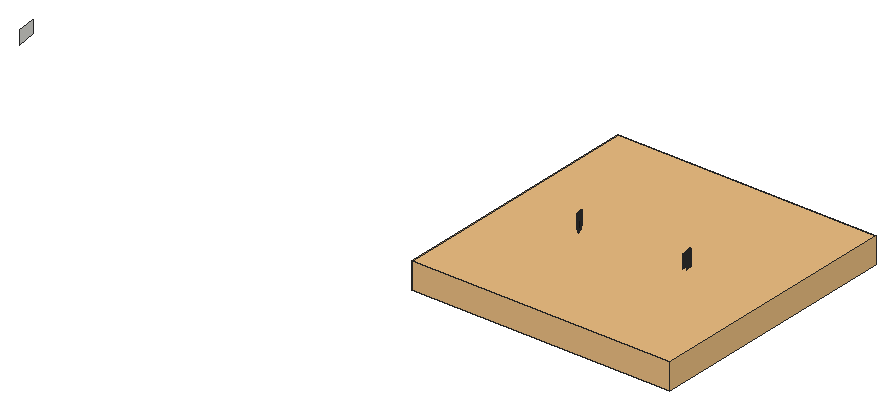
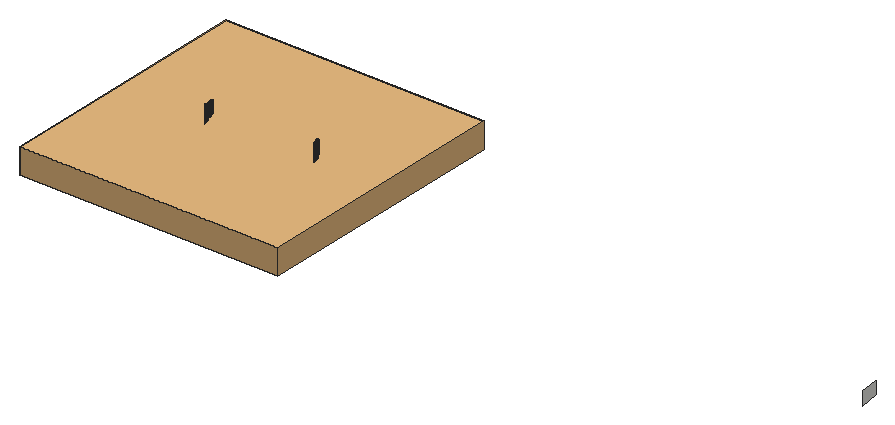
# SketchUp Ruby script. Lengths in inches.
U = 1.inch
M = Sketchup.active_model
def pt(a) = Geom::Point3d.new(a.map { |v| v * U })
def face(e, loops, mat)
  f = e.add_face(loops[0].map { |a| pt(a) })
  loops[1..].each { |l| e.add_face(l.map { |a| pt(a) }).erase! }
  f.material = f.back_material = mat if mat
  f
end
# faces: each face lists its corners as indices into pts; further lists are holes
def faces(e, pts, list, mat = nil) = list.each { |f| face(e, (f[0].is_a?(Array) ? f : [f]).map { |l| l.map { |i| pts[i] } }, mat) }
# xy, xz, yz: faces in a plane at the given z, y or x. An outline is a flat list of corners, or four numbers for a rectangle; further outlines are holes
def ring(l) = l.size == 4 ? [[l[0], l[1]], [l[2], l[1]], [l[2], l[3]], [l[0], l[3]]] : l.each_slice(2).to_a
def flat(e, list, mat, &to3) = list.each { |f| face(e, (f[0].is_a?(Array) ? f : [f]).map { |l| ring(l).map { |u, v| to3.(u, v) } }, mat) }
def xy(e, z, list, mat = nil) = flat(e, list, mat) { |x, y| [x, y, z] }
def xz(e, y, list, mat = nil) = flat(e, list, mat) { |x, z| [x, y, z] }
def yz(e, x, list, mat = nil) = flat(e, list, mat) { |y, z| [x, y, z] }
def lines(e, pts, list) = list.each { |a, b| e.add_line(pt(pts[a]), pt(pts[b])) }
# prism: a flat outline (further loops are holes) pulled along v
def prism(e, loops, v, mat = nil)
  f = face(e, loops, mat); d = Geom::Vector3d.new(v.map { |x| x * U })
  f.pushpull(f.normal.samedirection?(d) ? d.length : -d.length)
end
def box(e, o, s, mat = nil) = prism(e, [[o, [o[0] + s[0], o[1], o[2]], [o[0] + s[0], o[1] + s[1], o[2]], [o[0], o[1] + s[1], o[2]]]], [0, 0, s[2]], mat)
def at(x, y, z, deg = 0) = Geom::Transformation.translation(pt([x, y, z])) * Geom::Transformation.rotation(ORIGIN, Z_AXIS, deg.degrees)
def axes(o, x, y, z) = Geom::Transformation.new([*x, 0, *y, 0, *z, 0, *pt(o).to_a, 1])
def part(name) = M.definitions.add(name)
# library, detail: a bought-in or finely detailed component or shape, given as its bounding box
def library(name, o, s) = part(name).tap { |d| box(d.entities, o, s) }
def detail(e, o, s) = box(e.add_group.entities, o, s)
def put(e, d, t, mat = nil) = e.add_instance(d, t).tap { |i| i.material = mat if mat }
def group(e, t, mat = nil) = e.add_group.tap { |g| g.transformation = t; g.material = mat if mat }.entities
root = M.entities
M.materials.add("Marble_07_1K").color = [36, 34, 36]
c1 = library("Group\#6",[0,0,0],[120.09,120.15,12])
xy(root,0,[[365.49,782.54,365.54,782.54,365.51,782.62,365.5,782.67,365.45,782.75,365.4375,782.78,365.42,782.83,365.39,782.89,365.375,782.93,365.36,782.98,365.35,783.03,365.36,783.08,365.36,783.14,365.38,783.1875,365.4,783.24,365.42,783.28,365.44,783.34,365.47,783.39,365.55,783.55,365.64,783.7,365.65,783.76,365.65,783.81,365.64,783.875,365.63,783.92,365.61,783.98,365.59,784.03,365.56,784.07,365.52,784.14,365.49,784.18,365.47,784.22,365.43,784.26,365.39,784.33,365.35,784.38,365.32,784.41,365.26,784.5,365.23,784.55,365.21,784.59,365.18,784.64,365.2,784.74,365.19,784.79,365.21,784.83,365.21,784.88,365.2,784.92,365.22,784.97,365.22,785.03,365.23,785.09,365.23,785.24,365.22,785.29,365.2,785.35,365.19,785.39,365.18,785.4375,365.17,785.49,365.15,785.54,365.13,785.64,365.11,785.7,365.09,785.78,365.07,785.84,365.04,785.89,365.02,785.93,364.99,785.97,364.96,786.02,364.95,786.07,364.95,786.18,364.99,786.28,365.02,786.33,365.03,786.37,365.06,786.41,365.09,786.44,365.12,786.48,365.14,786.52,365.14,786.63,365.13,786.6875,365.1,786.74,365.08,786.78,365.05,786.83,365.01,786.87,364.97,786.92,364.9375,786.95,364.9,786.99,364.86,787.05,364.83,787.07,364.79,787.11,364.75,787.17,364.71,787.21,364.6875,787.25,364.66,787.29,364.61,787.34,364.59,787.38,364.58,787.42,364.55,787.46,364.53,787.56,364.52,787.6,364.52,787.64,364.51,787.69,364.52,787.73,364.52,787.78,364.53,787.83,364.52,787.87,364.53,787.93,364.54,787.98,364.56,788.02,364.58,788.0625,364.57,788.11,364.59,788.16,364.59,788.2,364.58,788.27,364.57,788.3,364.57,788.44,364.53,788.54,364.5,788.59,364.49,788.63,364.46,788.66,364.44,788.72,364.41,788.75,364.38,788.79,364.36,788.84,364.3,788.92,364.27,788.97,364.24,789.01,364.23,789.05,364.21,789.1,364.2,789.15,364.19,789.19,364.17,789.24,364.16,789.28,364.15,789.33,364.14,789.37,364.12,789.42,364.08,789.47,364.06,789.52,364.03,789.55,364,789.59,363.96,789.62,363.9,789.68,363.86,789.71,363.71,789.75,363.68,789.67,363.71,789.54,363.72,789.52,363.72,789.46,363.74,789.38,363.75,789.33,363.77,789.28,363.79,789.18,363.81,789.125,363.83,789.08,363.84,789.04,363.86,788.98,363.88,788.9375,363.89,788.9,363.9,788.85,363.91,788.81,363.93,788.77,363.9375,788.73,363.96,788.6875,363.96,788.64,363.97,788.6,363.99,788.55,363.98,788.51,364,788.41,364,788.36,363.99,788.3,363.99,788.24,363.98,788.1875,363.99,788.14,363.97,788.1,363.98,788.04,363.97,787.97,363.97,787.93,363.99,787.875,363.99,787.83,364.01,787.78,364.03,787.72,364.04,787.68,364.06,787.625,364.08,787.58,364.1,787.52,364.12,787.49,364.13,787.44,364.16,787.375,364.17,787.33,364.2,787.28,364.21,787.24,364.23,787.18,364.24,787.14,364.26,787.09,364.28,787.05,364.3,787,364.33,786.96,364.34,786.92,364.35,786.87,364.375,786.83,364.39,786.75,364.38,786.71,364.37,786.66,364.37,786.62,364.36,786.57,364.35,786.51,364.33,786.46,364.32,786.41,364.3125,786.35,364.3,786.28,364.29,786.21,364.3,786.14,364.3,786.04,364.33,785.99,364.36,785.92,364.375,785.88,364.43,785.77,364.45,785.71,364.49,785.66,364.52,785.61,364.55,785.5625,364.57,785.52,364.6,785.48,364.62,785.4375,364.65,785.39,364.74,785.24,364.78,785.2,364.8,785.16,364.83,785.11,364.88,785.01,364.87,784.95,364.85,784.9,364.84,784.86,364.82,784.8125,364.79,784.76,364.77,784.71,364.75,784.67,364.72,784.625,364.72,784.58,364.7,784.53,364.67,784.48,364.67,784.43,364.66,784.38,364.66,784.33,364.67,784.26,364.67,784.2,364.66,784.16,364.67,784.08,364.68,784.04,364.68,783.97,364.7,783.89,364.7,783.85,364.71,783.8,364.73,783.74,364.76,783.68,364.77,783.64,364.83,783.52,364.85,783.47,364.88,783.42,364.92,783.3,364.93,783.26,364.93,783.16,364.92,783.12,364.9,783.07,364.875,783.01,364.86,782.97,364.83,782.92,364.81,782.88,364.79,782.83,364.76,782.79,364.76,782.74,364.85,782.65,364.91,782.65,365.01,782.63,365.1,782.61,365.19,782.6,365.29,782.58,365.375,782.55,365.4375,782.55]],"Marble_07_1K")
yz(root,315.28,[[785.23,0,785.29,18]],"Marble_07_1K")
yz(root,315.29,[[785.15,0,785.19,18]],"Marble_07_1K")
yz(root,315.46,[[784.59,0,784.63,18]],"Marble_07_1K")
yz(root,315.52,[[784.37,0,784.41,18]],"Marble_07_1K")
yz(root,315.53,[[783.7,0,783.75,18]],"Marble_07_1K")
yz(root,315.54,[[783.91,0,783.96,18],[783.96,0,784.02,18],[784.29,0,784.33,18]],"Marble_07_1K")
yz(root,315.55,[[784.07,0,784.14,18],[784.14,0,784.1875,18],[784.1875,0,784.23,18]],"Marble_07_1K")
yz(root,315.68,[[783.21,0,783.26,18]],"Marble_07_1K")
yz(root,315.75,[[784.92,0,784.97,18]],"Marble_07_1K")
yz(root,315.88,[[782.1875,0,782.23,18]],"Marble_07_1K")
yz(root,315.93,[[782.39,0,782.4375,18]],"Marble_07_1K")
yz(root,316.07,[[783.42,0,783.46,18]],"Marble_07_1K")
yz(root,316.08,[[783.51,0,783.55,18],[783.55,0,783.6,18],[783.6,0,783.65,18]],"Marble_07_1K")
yz(root,316.1,[[783.24,0,783.29,18]],"Marble_07_1K")
yz(root,316.13,[[784.08,0,784.13,18]],"Marble_07_1K")
yz(root,316.14,[[783.93,0,783.97,18],[783.97,0,784.04,18]],"Marble_07_1K")
yz(root,316.7,[[782.3,0,782.37,18],[782.37,0,782.41,18]],"Marble_07_1K")
yz(root,364.3,[[786.04,0,786.09,18],[786.09,0,786.14,18]],"Marble_07_1K")
yz(root,364.37,[[786.62,0,786.66,18]],"Marble_07_1K")
yz(root,364.52,[[787.6,0,787.64,18],[787.73,0,787.78,18]],"Marble_07_1K")
yz(root,364.66,[[784.33,0,784.38,18]],"Marble_07_1K")
yz(root,364.67,[[784.2,0,784.26,18],[784.43,0,784.48,18]],"Marble_07_1K")
yz(root,364.68,[[783.97,0,784.04,18]],"Marble_07_1K")
yz(root,364.7,[[783.85,0,783.89,18]],"Marble_07_1K")
yz(root,364.72,[[784.58,0,784.625,18]],"Marble_07_1K")
yz(root,364.76,[[782.74,0,782.79,18]],"Marble_07_1K")
p = [[58.16,787.52,0],[59.15,778.47,0],[59.15,778.47,6],[58.16,787.52,6],[315.86,782.06,0],[315.86,782.06,18],
  [315.84,781.98,18],[315.84,781.98,0],[316.53,782,0],[316.53,782,18],[316.55,782.05,18],[316.55,782.05,0],
  [315.87,782.125,0],[315.87,782.125,18],[315.88,782.1875,0],[315.88,782.1875,18],[316.57,782.1,18],[316.57,782.1,0],
  [316.59,782.14,18],[316.59,782.14,0],[316.61,782.18,18],[316.61,782.18,0],[315.9,782.29,0],[315.9,782.29,18],
  [315.88,782.23,18],[315.88,782.23,0],[316.65,782.22,18],[316.65,782.22,0],[316.67,782.26,18],[316.67,782.26,0],
  [315.91,782.35,0],[315.91,782.35,18],[315.93,782.39,0],[315.93,782.39,18],[316.7,782.3,18],[316.7,782.3,0],
  [315.9375,782.48,0],[315.9375,782.48,18],[315.93,782.4375,18],[315.93,782.4375,0],[316.7,782.41,0],[316.7,782.41,18],
  [316.68,782.46,18],[316.68,782.46,0],[315.94,782.52,0],[315.94,782.52,18],[315.93,782.6,0],[315.93,782.6,18],
  [316.66,782.51,0],[316.66,782.51,18],[316.63,782.56,18],[316.63,782.56,0],[315.91,782.65,0],[315.91,782.65,18],
  [315.9,782.6875,0],[315.9,782.6875,18],[316.57,782.64,0],[316.57,782.64,18],[316.52,782.7,18],[316.52,782.7,0],
  [316.6,782.61,18],[316.6,782.61,0],[315.88,782.73,0],[315.88,782.73,18],[315.86,782.78,0],[315.86,782.78,18],
  [316.49,782.73,18],[316.49,782.73,0],[316.45,782.76,18],[316.45,782.76,0],[315.83,782.82,0],[315.83,782.82,18],
  [315.82,782.87,0],[315.82,782.87,18],[316.38,782.85,0],[316.38,782.85,18],[316.35,782.88,18],[316.35,782.88,0],
  [316.41,782.82,18],[316.41,782.82,0],[315.8,782.91,0],[315.8,782.91,18],[315.78,782.96,0],[315.78,782.96,18],
  [316.3,782.94,18],[316.3,782.94,0],[316.27,782.99,18],[316.27,782.99,0],[315.76,783.01,0],[315.76,783.01,18],
  [315.75,783.05,0],[315.75,783.05,18],[316.25,783.02,18],[316.25,783.02,0],[316.21,783.06,18],[316.21,783.06,0],
  [315.73,783.1,0],[315.73,783.1,18],[315.71,783.15,0],[315.71,783.15,18],[315.68,783.21,0],[315.68,783.21,18],
  [316.17,783.12,0],[316.17,783.12,18],[316.15,783.15,18],[316.15,783.15,0],[316.13,783.19,18],[316.13,783.19,0],
  [316.1,783.24,18],[316.1,783.24,0],[315.64,783.35,0],[315.64,783.35,18],[315.66,783.29,18],[315.66,783.29,0],
  [315.68,783.26,18],[315.68,783.26,0],[316.1,783.29,0],[316.1,783.29,18],[316.09,783.33,18],[316.09,783.33,0],
  [316.08,783.375,18],[316.08,783.375,0],[315.61,783.4,0],[315.61,783.4,18],[315.6,783.46,0],[315.6,783.46,18],
  [316.07,783.42,18],[316.07,783.42,0],[315.55,783.6,0],[315.55,783.6,18],[315.57,783.55,18],[315.57,783.55,0],
  [315.59,783.5,0],[315.59,783.5,18],[316.07,783.46,0],[316.07,783.46,18],[316.08,783.51,18],[316.08,783.51,0],
  [315.54,783.65,0],[315.54,783.65,18],[315.53,783.7,0],[315.53,783.7,18],[316.08,783.65,0],[316.08,783.65,18],
  [316.09,783.71,18],[316.09,783.71,0],[364.76,783.68,0],[364.76,783.68,18],[364.77,783.64,18],[364.77,783.64,0],
  [315.54,783.81,0],[315.54,783.81,18],[315.53,783.75,18],[315.53,783.75,0],[316.1,783.75,18],[316.1,783.75,0],
  [364.73,783.74,0],[364.73,783.74,18],[364.71,783.8,0],[364.71,783.8,18],[315.53,783.87,0],[315.53,783.87,18],
  [316.12,783.79,18],[316.12,783.79,0],[316.13,783.84,18],[316.13,783.84,0],[316.125,783.89,18],[316.125,783.89,0],
  [364.7,783.85,0],[364.7,783.85,18],[315.54,783.91,0],[315.54,783.91,18],[316.14,783.93,18],[316.14,783.93,0],
  [364.68,783.97,0],[364.68,783.97,18],[364.7,783.89,18],[364.7,783.89,0],[315.55,784.07,0],[315.55,784.07,18],
  [315.54,784.02,18],[315.54,784.02,0],[316.14,784.04,0],[316.14,784.04,18],[316.13,784.08,18],[316.13,784.08,0],
  [364.67,784.08,0],[364.67,784.08,18],[364.68,784.04,18],[364.68,784.04,0],[316.13,784.13,0],[316.13,784.13,18],
  [316.125,784.17,18],[316.125,784.17,0],[364.66,784.16,0],[364.66,784.16,18],[315.54,784.29,0],[315.54,784.29,18],
  [315.55,784.23,18],[315.55,784.23,0],[316.12,784.22,18],[316.12,784.22,0],[316.1,784.27,18],[316.1,784.27,0],
  [364.67,784.2,0],[364.67,784.2,18],[315.52,784.37,0],[315.52,784.37,18],[315.54,784.33,18],[315.54,784.33,0],
  [316.08,784.31,18],[316.08,784.31,0],[316.06,784.36,18],[316.06,784.36,0],[364.66,784.33,0],[364.66,784.33,18],
  [364.67,784.26,18],[364.67,784.26,0],[315.51,784.46,0],[315.51,784.46,18],[315.52,784.41,18],[315.52,784.41,0],
  [316.05,784.4,18],[316.05,784.4,0],[316.02,784.4375,18],[316.02,784.4375,0],[316,784.49,18],[316,784.49,0],
  [364.67,784.43,0],[364.67,784.43,18],[364.66,784.38,18],[364.66,784.38,0],[315.49,784.51,0],[315.49,784.51,18],
  [315.48,784.55,0],[315.48,784.55,18],[315.46,784.59,0],[315.46,784.59,18],[315.97,784.53,0],[315.97,784.53,18],
  [315.9375,784.57,18],[315.9375,784.57,0],[364.7,784.53,0],[364.7,784.53,18],[364.67,784.48,18],[364.67,784.48,0],
  [364.72,784.58,0],[364.72,784.58,18],[315.45,784.67,0],[315.45,784.67,18],[315.46,784.63,18],[315.46,784.63,0],
  [315.91,784.62,18],[315.91,784.62,0],[315.88,784.66,18],[315.88,784.66,0],[364.75,784.67,0],[364.75,784.67,18],
  [364.72,784.625,18],[364.72,784.625,0],[315.4375,784.71,0],[315.4375,784.71,18],[315.41,784.76,0],[315.41,784.76,18],
  [315.85,784.7,0],[315.85,784.7,18],[315.83,784.75,18],[315.83,784.75,0],[315.8,784.79,18],[315.8,784.79,0],
  [364.77,784.71,0],[364.77,784.71,18],[315.4,784.8125,0],[315.4,784.8125,18],[315.39,784.86,0],[315.39,784.86,18],
  [315.78,784.83,18],[315.78,784.83,0],[315.76,784.875,18],[315.76,784.875,0],[315.35,784.96,0],[315.35,784.96,18],
  [315.36,784.9,18],[315.36,784.9,0],[315.75,784.92,18],[315.75,784.92,0],[315.33,785.01,0],[315.33,785.01,18],
  [315.32,785.05,0],[315.32,785.05,18],[315.31,785.11,0],[315.31,785.11,18],[315.75,784.97,0],[315.75,784.97,18],
  [315.73,785.02,18],[315.73,785.02,0],[315.72,785.06,18],[315.72,785.06,0],[315.29,785.15,0],[315.29,785.15,18],
  [315.7,785.1,18],[315.7,785.1,0],[315.69,785.15,18],[315.69,785.15,0],[315.67,785.19,18],[315.67,785.19,0],
  [315.28,785.23,0],[315.28,785.23,18],[315.29,785.19,18],[315.29,785.19,0],[315.64,785.24,18],[315.64,785.24,0],
  [315.62,785.29,18],[315.62,785.29,0],[364.74,785.24,0],[364.74,785.24,18],[364.78,785.2,18],[364.78,785.2,0],
  [364.71,785.29,0],[364.71,785.29,18],[315.24,785.44,0],[315.24,785.44,18],[315.27,785.32,18],[315.27,785.32,0],
  [315.28,785.29,18],[315.28,785.29,0],[315.58,785.33,18],[315.58,785.33,0],[315.55,785.36,18],[315.55,785.36,0],
  [364.65,785.39,0],[364.65,785.39,18],[364.68,785.34,18],[364.68,785.34,0],[315.26,785.53,0],[315.26,785.53,18],
  [315.45,785.45,0],[315.45,785.45,18],[315.42,785.48,18],[315.42,785.48,0],[315.52,785.39,18],[315.52,785.39,0],
  [315.49,785.42,18],[315.49,785.42,0],[364.62,785.4375,0],[364.62,785.4375,18],[364.6,785.48,0],[364.6,785.48,18],
  [364.55,785.5625,0],[364.55,785.5625,18],[364.57,785.52,18],[364.57,785.52,0],[364.52,785.61,0],[364.52,785.61,18],
  [364.49,785.66,0],[364.49,785.66,18],[364.43,785.77,0],[364.43,785.77,18],[364.45,785.71,18],[364.45,785.71,0],
  [364.4,785.83,0],[364.4,785.83,18],[364.375,785.88,0],[364.375,785.88,18],[364.33,785.99,0],[364.33,785.99,18],
  [364.36,785.92,18],[364.36,785.92,0],[364.3,786.04,0],[364.3,786.04,18],[364.29,786.21,0],[364.29,786.21,18],
  [364.3,786.14,18],[364.3,786.14,0],[364.3,786.28,0],[364.3,786.28,18],[364.3125,786.35,0],[364.3125,786.35,18],
  [364.32,786.41,0],[364.32,786.41,18],[364.33,786.46,0],[364.33,786.46,18],[364.35,786.51,0],[364.35,786.51,18],
  [364.36,786.57,0],[364.36,786.57,18],[364.37,786.62,0],[364.37,786.62,18],[364.38,786.71,0],[364.38,786.71,18],
  [364.37,786.66,18],[364.37,786.66,0],[364.39,786.75,0],[364.39,786.75,18],[364.375,786.83,0],[364.375,786.83,18],
  [364.35,786.87,0],[364.35,786.87,18],[364.34,786.92,0],[364.34,786.92,18],[364.33,786.96,0],[364.33,786.96,18],
  [364.3,787,0],[364.3,787,18],[364.28,787.05,0],[364.28,787.05,18],[364.26,787.09,0],[364.26,787.09,18],
  [364.24,787.14,0],[364.24,787.14,18],[364.23,787.18,0],[364.23,787.18,18],[364.21,787.24,0],[364.21,787.24,18],
  [364.2,787.28,0],[364.2,787.28,18],[364.75,787.17,0],[364.75,787.17,18],[364.71,787.21,18],[364.71,787.21,0],
  [364.6875,787.25,18],[364.6875,787.25,0],[364.66,787.29,18],[364.66,787.29,0],[364.17,787.33,0],[364.17,787.33,18],
  [364.16,787.375,0],[364.16,787.375,18],[364.61,787.34,18],[364.61,787.34,0],[364.59,787.38,18],[364.59,787.38,0],
  [364.13,787.44,0],[364.13,787.44,18],[364.12,787.49,0],[364.12,787.49,18],[364.58,787.42,0],[364.58,787.42,18],
  [364.55,787.46,18],[364.55,787.46,0],[364.1,787.52,0],[364.1,787.52,18],[364.08,787.58,0],[364.08,787.58,18],
  [364.54,787.51,18],[364.54,787.51,0],[364.53,787.56,18],[364.53,787.56,0],[364.04,787.68,0],[364.04,787.68,18],
  [364.06,787.625,18],[364.06,787.625,0],[364.52,787.6,18],[364.52,787.6,0],[364.52,787.64,0],[364.52,787.64,18],
  [364.51,787.69,18],[364.51,787.69,0],[364.03,787.72,0],[364.03,787.72,18],[364.01,787.78,0],[364.01,787.78,18],
  [364.52,787.73,18],[364.52,787.73,0],[363.99,787.83,0],[363.99,787.83,18],[284.28,725.46,0],[284.28,845.62,0]]
faces(root,p,[[0,1,2,3]])
faces(root,p,[[4,5,6,7],[8,9,10,11],[12,13,5,4],[14,15,13,12],[11,10,16,17],[17,16,18,19],[19,18,20,21],[22,23,24,25],
  [21,20,26,27],[27,26,28,29],[30,31,23,22],[32,33,31,30],[29,28,34,35],[36,37,38,39],[40,41,42,43],[44,45,37,36],
  [46,47,45,44],[48,49,50,51],[43,42,49,48],[52,53,47,46],[54,55,53,52],[56,57,58,59],[51,50,60,61],[61,60,57,56],
  [62,63,55,54],[64,65,63,62],[59,58,66,67],[67,66,68,69],[70,71,65,64],[72,73,71,70],[74,75,76,77],[69,68,78,79],
  [79,78,75,74],[80,81,73,72],[82,83,81,80],[77,76,84,85],[85,84,86,87],[88,89,83,82],[90,91,89,88],[87,86,92,93],
  [93,92,94,95],[96,97,91,90],[98,99,97,96],[100,101,99,98],[102,103,104,105],[95,94,103,102],[105,104,106,107],[107,106,108,109],
  [110,111,112,113],[113,112,114,115],[116,117,118,119],[119,118,120,121],[122,123,111,110],[124,125,123,122],[121,120,126,127],[128,129,130,131],
  [132,133,125,124],[131,130,133,132],[134,135,136,137],[138,139,129,128],[140,141,139,138],[142,143,144,145],[146,147,148,149],[150,151,152,153],
  [145,144,154,155],[156,157,147,146],[158,159,157,156],[160,161,151,150],[155,154,162,163],[163,162,164,165],[165,164,166,167],[168,169,159,158],
  [170,171,161,160],[167,166,172,173],[174,175,176,177],[178,179,180,181],[182,183,184,185],[186,187,188,189],[190,191,192,193],[194,195,187,186],
  [196,197,198,199],[193,192,200,201],[201,200,202,203],[204,205,195,194],[206,207,208,209],[203,202,210,211],[211,210,212,213],[214,215,216,217],
  [218,219,220,221],[213,212,222,223],[223,222,224,225],[225,224,226,227],[228,229,230,231],[232,233,219,218],[234,235,233,232],[236,237,235,234],
  [238,239,240,241],[227,226,239,238],[242,243,244,245],[246,247,243,242],[248,249,250,251],[241,240,252,253],[253,252,254,255],[256,257,258,259],
  [260,261,249,248],[262,263,261,260],[264,265,266,267],[267,266,268,269],[255,254,265,264],[270,271,257,256],[272,273,263,262],[274,275,273,272],
  [269,268,276,277],[277,276,278,279],[280,281,282,283],[283,282,275,274],[279,278,284,285],[286,287,281,280],[288,289,287,286],[290,291,289,288],
  [292,293,294,295],[295,294,296,297],[298,299,291,290],[297,296,300,301],[301,300,302,303],[303,302,304,305],[306,307,308,309],[305,304,310,311],
  [311,310,312,313],[314,315,316,317],[318,319,315,314],[320,321,322,323],[323,322,324,325],[313,312,326,327],[327,326,328,329],[330,331,332,333],
  [333,332,319,318],[334,335,321,320],[336,337,338,339],[329,328,340,341],[341,340,342,343],[343,342,337,336],[344,345,331,330],[346,347,345,344],
  [339,338,335,334],[348,349,350,351],[351,350,347,346],[352,353,349,348],[354,355,353,352],[356,357,358,359],[359,358,355,354],[360,361,357,356],
  [362,363,361,360],[364,365,366,367],[367,366,363,362],[368,369,365,364],[370,371,372,373],[374,375,371,370],[376,377,375,374],[378,379,377,376],
  [380,381,379,378],[382,383,381,380],[384,385,383,382],[386,387,385,384],[388,389,390,391],[392,393,389,388],[394,395,393,392],[396,397,395,394],
  [398,399,397,396],[400,401,399,398],[402,403,401,400],[404,405,403,402],[406,407,405,404],[408,409,407,406],[410,411,409,408],[412,413,411,410],
  [414,415,413,412],[416,417,418,419],[419,418,420,421],[421,420,422,423],[424,425,415,414],[426,427,425,424],[423,422,428,429],[429,428,430,431],
  [432,433,427,426],[434,435,433,432],[436,437,438,439],[431,430,437,436],[440,441,435,434],[442,443,441,440],[439,438,444,445],[445,444,446,447],
  [448,449,450,451],[451,450,443,442],[447,446,452,453],[454,455,456,457],[458,459,449,448],[460,461,459,458],[457,456,462,463],[464,465,461,460]],"Marble_07_1K")
lines(root,p,[[466,467]])
put(root,c1,at(284.28,725.46,0))
